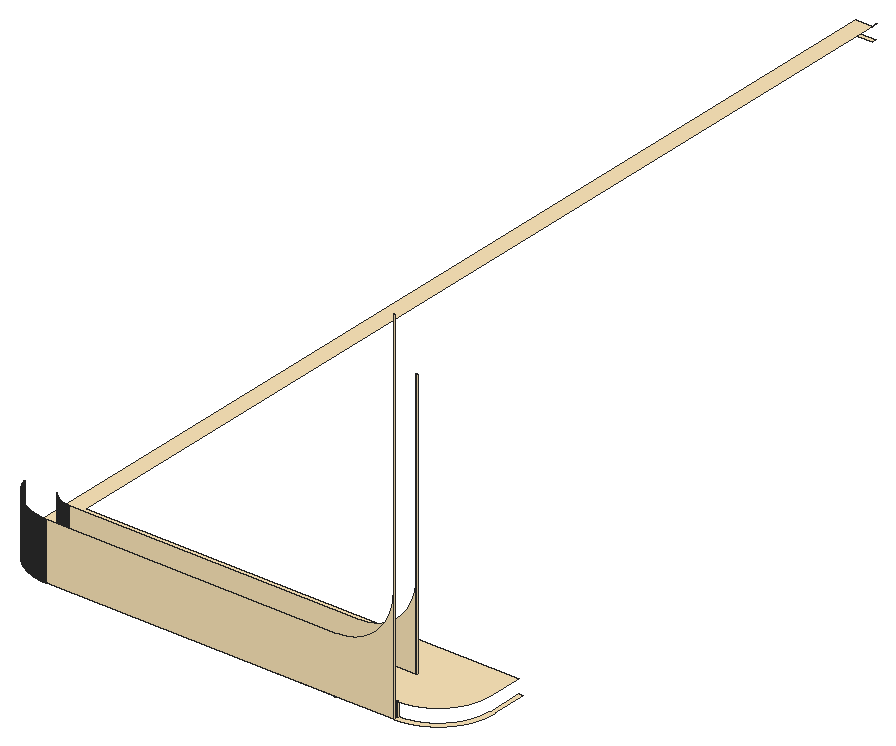
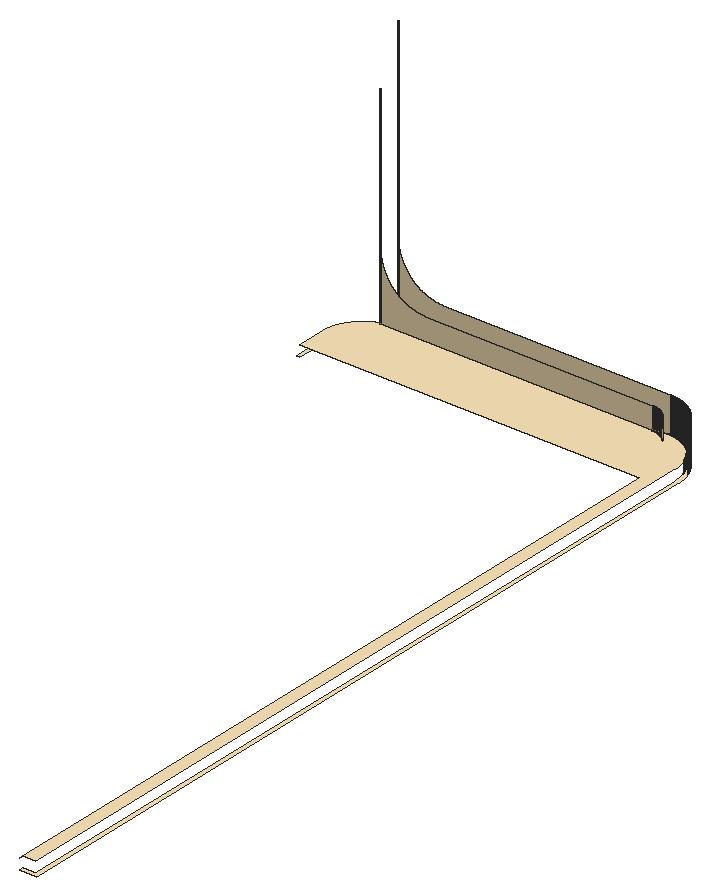
# SketchUp Ruby script. Lengths in inches.
U = 1.inch
M = Sketchup.active_model
def pt(a) = Geom::Point3d.new(a.map { |v| v * U })
def face(e, loops, mat)
  f = e.add_face(loops[0].map { |a| pt(a) })
  loops[1..].each { |l| e.add_face(l.map { |a| pt(a) }).erase! }
  f.material = f.back_material = mat if mat
  f
end
# faces: each face lists its corners as indices into pts; further lists are holes
def faces(e, pts, list, mat = nil) = list.each { |f| face(e, (f[0].is_a?(Array) ? f : [f]).map { |l| l.map { |i| pts[i] } }, mat) }
# xy, xz, yz: faces in a plane at the given z, y or x. An outline is a flat list of corners, or four numbers for a rectangle; further outlines are holes
def ring(l) = l.size == 4 ? [[l[0], l[1]], [l[2], l[1]], [l[2], l[3]], [l[0], l[3]]] : l.each_slice(2).to_a
def flat(e, list, mat, &to3) = list.each { |f| face(e, (f[0].is_a?(Array) ? f : [f]).map { |l| ring(l).map { |u, v| to3.(u, v) } }, mat) }
def xy(e, z, list, mat = nil) = flat(e, list, mat) { |x, y| [x, y, z] }
def xz(e, y, list, mat = nil) = flat(e, list, mat) { |x, z| [x, y, z] }
def yz(e, x, list, mat = nil) = flat(e, list, mat) { |y, z| [x, y, z] }
def lines(e, pts, list) = list.each { |a, b| e.add_line(pt(pts[a]), pt(pts[b])) }
# prism: a flat outline (further loops are holes) pulled along v
def prism(e, loops, v, mat = nil)
  f = face(e, loops, mat); d = Geom::Vector3d.new(v.map { |x| x * U })
  f.pushpull(f.normal.samedirection?(d) ? d.length : -d.length)
end
def box(e, o, s, mat = nil) = prism(e, [[o, [o[0] + s[0], o[1], o[2]], [o[0] + s[0], o[1] + s[1], o[2]], [o[0], o[1] + s[1], o[2]]]], [0, 0, s[2]], mat)
def at(x, y, z, deg = 0) = Geom::Transformation.translation(pt([x, y, z])) * Geom::Transformation.rotation(ORIGIN, Z_AXIS, deg.degrees)
def axes(o, x, y, z) = Geom::Transformation.new([*x, 0, *y, 0, *z, 0, *pt(o).to_a, 1])
def part(name) = M.definitions.add(name)
# library, detail: a bought-in or finely detailed component or shape, given as its bounding box
def library(name, o, s) = part(name).tap { |d| box(d.entities, o, s) }
def detail(e, o, s) = box(e.add_group.entities, o, s)
def put(e, d, t, mat = nil) = e.add_instance(d, t).tap { |i| i.material = mat if mat }
def group(e, t, mat = nil) = e.add_group.tap { |g| g.transformation = t; g.material = mat if mat }.entities
root = M.entities
M.materials.add("1026 AP 7946 SUNNY SIDE UP").color = [254, 231, 186]
xy(root,120,[[153,215,29.765,215.001,29.529,215.005,29.294,215.01,29.059,215.018,28.824,215.029,28.589,215.041,28.354,215.056,28.119,215.074,27.885,215.093,27.65,215.115,27.416,215.139,27.182,215.166,26.949,215.195,26.715,215.226,26.483,215.259,26.25,215.295,26.018,215.333,25.786,215.373,25.554,215.415,25.323,215.46,25.093,215.507,24.862,215.556,24.633,215.608,24.404,215.661,24.175,215.717,23.947,215.776,23.72,215.836,23.493,215.899,23.267,215.964,23.041,216.031,22.816,216.1,22.592,216.172,22.368,216.246,22.146,216.321,21.924,216.4,21.702,216.48,21.482,216.562,21.262,216.647,21.044,216.734,20.826,216.823,20.609,216.914,20.392,217.007,20.177,217.102,19.963,217.199,19.75,217.299,19.537,217.4,19.326,217.504,19.116,217.61,18.907,217.717,18.698,217.827,18.491,217.939,18.285,218.053,18.081,218.169,17.877,218.287,17.674,218.407,17.473,218.528,17.273,218.652,17.074,218.778,16.876,218.906,16.68,219.035,16.485,219.167,16.291,219.3,16.098,219.436,15.907,219.573,15.717,219.712,15.529,219.853,15.342,219.996,15.156,220.141,14.972,220.287,14.789,220.435,14.608,220.585,14.428,220.737,14.25,220.891,14.073,221.046,13.898,221.203,13.724,221.362,13.552,221.522,13.381,221.684,13.212,221.848,13.045,222.014,12.879,222.181,12.715,222.349,12.552,222.52,12.392,222.692,12.233,222.865,12.075,223.04,11.92,223.217,11.766,223.395,11.614,223.574,11.463,223.755,11.315,223.9375,11.168,224.122,11.023,224.307,10.88,224.494,10.738,224.682,10.599,224.872,10.461,225.0625,10.325,225.255,10.192,225.448,10.06,225.643,9.93,225.839,9.802,226.037,9.675,226.235,9.551,226.435,9.429,226.637,9.309,226.839,9.19,227.042,9.074,227.247,8.96,227.453,8.848,227.66,8.738,227.868,8.629,228.077,8.523,228.287,8.419,228.498,8.317,228.71,8.218,228.923,8.12,229.137,8.024,229.352,7.931,229.568,7.839,229.785,7.75,230.003,7.663,230.221,7.578,230.441,7.495,230.661,7.414,230.882,7.336,231.104,7.259,231.327,7.185,231.55,7.113,231.774,7.043,231.999,6.976,232.224,6.91,232.45,6.847,232.677,6.786,232.904,6.728,233.132,6.671,233.361,6.617,233.59,6.565,233.819,6.516,234.049,6.468,234.28,6.423,234.511,6.38,234.742,6.34,234.974,6.301,235.206,6.265,235.439,6.231,235.672,6.2,235.905,6.171,236.138,6.144,236.372,6.119,236.606,6.097,236.841,6.077,237.075,6.059,237.31,6.044,237.545,6.031,237.78,6.02,238.015,6.011,238.25,6.005,238.485,6.001,238.72,5.999,238.956,6,239,6,674,15,674,15,672,8,672,8,238.989,7.999,238.96,8.001,238.744,8.005,238.528,8.01,238.3125,8.018,238.097,8.028,237.881,8.04,237.666,8.054,237.451,8.07,237.236,8.089,237.021,8.109,236.806,8.132,236.591,8.156,236.377,8.183,236.163,8.212,235.949,8.243,235.736,8.276,235.522,8.311,235.31,8.348,235.097,8.388,234.885,8.429,234.673,8.473,234.462,8.518,234.251,8.566,234.041,8.615,233.831,8.667,233.621,8.721,233.412,8.777,233.204,8.835,232.996,8.894,232.789,8.956,232.582,9.02,232.376,9.086,232.171,9.154,231.966,9.224,231.762,9.296,231.559,9.37,231.356,9.446,231.154,9.524,230.953,9.604,230.752,9.686,230.553,9.77,230.354,9.855,230.156,9.943,229.959,10.033,229.763,10.124,229.567,10.218,229.373,10.313,229.179,10.41,228.987,10.509,228.795,10.61,228.605,10.713,228.415,10.818,228.226,10.925,228.039,11.033,227.852,11.143,227.667,11.255,227.482,11.369,227.299,11.485,227.117,11.602,226.936,11.721,226.756,11.842,226.578,11.965,226.4,12.089,226.224,12.215,226.049,12.343,225.875,12.473,225.703,12.604,225.531,12.737,225.361,12.872,225.193,13.008,225.026,13.146,224.86,13.285,224.695,13.426,224.532,13.569,224.37,13.713,224.21,13.859,224.051,14.006,223.893,14.155,223.737,14.306,223.582,14.458,223.429,14.611,223.278,14.766,223.127,14.922,222.979,15.08,222.832,15.239,222.686,15.4,222.542,15.562,222.4,15.726,222.259,15.891,222.12,16.057,221.982,16.224,221.846,16.393,221.712,16.563,221.58,16.735,221.449,16.908,221.319,17.082,221.192,17.257,221.066,17.433,220.942,17.611,220.82,17.79,220.699,17.97,220.58,18.151,220.463,18.333,220.348,18.517,220.234,18.701,220.123,18.887,220.013,19.074,219.905,19.262,219.798,19.45,219.694,19.64,219.592,19.831,219.491,20.023,219.392,20.216,219.295,20.409,219.2,20.604,219.107,20.799,219.016,20.996,218.927,21.193,218.839,21.391,218.754,21.59,218.671,21.79,218.589,21.99,218.51,22.192,218.432,22.394,218.357,22.597,218.283,22.8,218.211,23.004,218.142,23.209,218.074,23.415,218.009,23.621,217.945,23.828,217.883,24.035,217.824,24.243,217.766,24.451,217.711,24.66,217.658,24.87,217.606,25.08,217.557,25.291,217.51,25.501,217.465,25.713,217.422,25.925,217.381,26.137,217.342,26.349,217.305,26.5625,217.27,26.776,217.237,26.989,217.207,27.203,217.178,27.417,217.152,27.631,217.128,27.846,217.106,28.061,217.086,28.276,217.068,28.491,217.052,28.706,217.038,28.922,217.026,29.137,217.017,29.353,217.01,29.569,217.004,29.784,217.001,153,217,177,217,177.23,217.001,177.461,217.005,177.691,217.011,177.921,217.019,178.151,217.03,178.381,217.043,178.611,217.059,178.841,217.077,179.07,217.098,179.3,217.121,179.529,217.146,179.757,217.173,179.986,217.204,180.214,217.236,180.442,217.271,180.669,217.308,180.896,217.348,181.122,217.39,181.348,217.434,181.574,217.481,181.799,217.53,182.024,217.581,182.248,217.635,182.471,217.691,182.694,217.75,182.916,217.81,183.138,217.874,183.359,217.939,183.579,218.007,183.798,218.077,184.017,218.149,184.235,218.224,184.452,218.301,184.669,218.38,184.884,218.461,185.099,218.545,185.3125,218.631,185.525,218.719,185.737,218.809,185.948,218.902,186.158,218.997,186.367,219.094,186.575,219.193,186.782,219.294,186.988,219.398,187.193,219.504,187.396,219.611,187.599,219.721,187.8,219.833,188,219.947,188.199,220.064,188.397,220.182,188.593,220.302,188.788,220.425,188.982,220.549,189.175,220.676,189.366,220.804,189.556,220.935,189.744,221.067,189.931,221.202,190.117,221.338,190.301,221.476,190.484,221.617,190.665,221.759,190.845,221.903,191.023,222.049,191.2,222.196,191.375,222.346,191.549,222.498,191.721,222.651,191.891,222.806,192.06,222.963,192.227,223.121,192.393,223.282,192.556,223.444,192.718,223.607,192.879,223.773,193.037,223.94,193.194,224.109,193.349,224.279,193.502,224.451,193.654,224.625,193.804,224.8,193.951,224.977,194.097,225.155,194.241,225.335,194.383,225.516,194.524,225.699,194.662,225.883,194.798,226.069,194.933,226.256,195.065,226.444,195.196,226.634,195.324,226.825,195.451,227.018,195.575,227.212,195.698,227.407,195.818,227.603,195.936,227.801,196.053,228,196.167,228.2,196.279,228.401,196.389,228.604,196.496,228.807,196.602,229.012,196.706,229.218,196.807,229.425,196.906,229.633,197.003,229.842,197.098,230.052,197.191,230.263,197.281,230.475,197.369,230.6875,197.455,230.901,197.539,231.116,197.62,231.331,197.699,231.548,197.776,231.765,197.851,231.983,197.923,232.202,197.993,232.421,198.061,232.641,198.126,232.862,198.19,233.084,198.25,233.306,198.309,233.529,198.365,233.752,198.419,233.976,198.47,234.201,198.519,234.426,198.566,234.652,198.61,234.878,198.652,235.104,198.692,235.331,198.729,235.558,198.764,235.786,198.796,236.014,198.827,236.243,198.854,236.471,198.879,236.7,198.902,236.93,198.923,237.159,198.941,237.389,198.957,237.619,198.97,237.849,198.981,238.079,198.989,238.309,198.995,238.539,198.999,238.77,199,239,199,254,201,254,201,239,200.999,238.749,200.995,238.497,200.988,238.246,200.979,237.995,200.967,237.744,200.953,237.493,200.936,237.242,200.916,236.992,200.893,236.741,200.869,236.491,200.841,236.242,200.811,235.992,200.778,235.743,200.743,235.494,200.705,235.246,200.664,234.998,200.621,234.75,200.575,234.503,200.527,234.256,200.476,234.01,200.422,233.765,200.366,233.52,200.307,233.275,200.246,233.031,200.182,232.788,200.116,232.546,200.047,232.304,199.976,232.063,199.902,231.823,199.825,231.584,199.746,231.345,199.665,231.107,199.581,230.87,199.495,230.634,199.406,230.399,199.315,230.165,199.221,229.932,199.125,229.7,199.026,229.468,198.925,229.238,198.822,229.009,198.716,228.781,198.608,228.554,198.497,228.329,198.384,228.104,198.269,227.881,198.151,227.659,198.031,227.438,197.909,227.218,197.785,227,197.658,226.783,197.529,226.567,197.397,226.353,197.264,226.14,197.128,225.929,196.99,225.719,196.85,225.51,196.708,225.303,196.563,225.097,196.416,224.893,196.268,224.691,196.117,224.49,195.964,224.29,195.809,224.092,195.652,223.896,195.492,223.702,195.331,223.509,195.168,223.318,195.003,223.129,194.835,222.941,194.666,222.755,194.495,222.571,194.322,222.389,194.147,222.208,193.971,222.029,193.792,221.853,193.611,221.678,193.429,221.505,193.245,221.334,193.059,221.165,192.871,220.997,192.682,220.832,192.491,220.669,192.298,220.508,192.104,220.348,191.908,220.191,191.71,220.036,191.51,219.883,191.309,219.732,191.107,219.584,190.903,219.437,190.697,219.292,190.49,219.15,190.281,219.01,190.071,218.872,189.86,218.736,189.647,218.603,189.433,218.471,189.217,218.342,189,218.215,188.782,218.091,188.562,217.969,188.341,217.849,188.119,217.731,187.896,217.616,187.671,217.503,187.446,217.392,187.219,217.284,186.991,217.178,186.762,217.075,186.532,216.974,186.3,216.875,186.068,216.779,185.835,216.685,185.601,216.594,185.366,216.505,185.13,216.419,184.893,216.335,184.655,216.254,184.416,216.175,184.177,216.098,183.937,216.024,183.696,215.953,183.454,215.884,183.212,215.818,182.969,215.754,182.725,215.693,182.48,215.634,182.235,215.578,181.99,215.524,181.744,215.473,181.497,215.425,181.25,215.379,181.002,215.336,180.754,215.295,180.506,215.257,180.257,215.222,180.008,215.189,179.758,215.159,179.509,215.131,179.259,215.107,179.008,215.084,178.758,215.064,178.507,215.047,178.256,215.033,178.005,215.021,177.754,215.012,177.503,215.005,177.251,215.001,177,215],[30,215,29.765,215.001,153,215]],"1026 AP 7946 SUNNY SIDE UP")
xy(root,126,[[153,217,29.784,217.001,29.569,217.004,29.353,217.01,29.137,217.017,28.922,217.026,28.706,217.038,28.491,217.052,28.276,217.068,28.061,217.086,27.846,217.106,27.631,217.128,27.417,217.152,27.203,217.178,26.989,217.207,26.776,217.237,26.5625,217.27,26.349,217.305,26.137,217.342,25.925,217.381,25.713,217.422,25.501,217.465,25.291,217.51,25.08,217.557,24.87,217.606,24.66,217.658,24.451,217.711,24.243,217.766,24.035,217.824,23.828,217.883,23.621,217.945,23.415,218.009,23.209,218.074,23.004,218.142,22.8,218.211,22.597,218.283,22.394,218.357,22.192,218.432,21.99,218.51,21.79,218.589,21.59,218.671,21.391,218.754,21.193,218.839,20.996,218.927,20.799,219.016,20.604,219.107,20.409,219.2,20.216,219.295,20.023,219.392,19.831,219.491,19.64,219.592,19.45,219.694,19.262,219.798,19.074,219.905,18.887,220.013,18.701,220.123,18.517,220.234,18.333,220.348,18.151,220.463,17.97,220.58,17.79,220.699,17.611,220.82,17.433,220.942,17.257,221.066,17.082,221.192,16.908,221.319,16.735,221.449,16.563,221.58,16.393,221.712,16.224,221.846,16.057,221.982,15.891,222.12,15.726,222.259,15.562,222.4,15.4,222.542,15.239,222.686,15.08,222.832,14.922,222.979,14.766,223.127,14.611,223.278,14.458,223.429,14.306,223.582,14.155,223.737,14.006,223.893,13.859,224.051,13.713,224.21,13.569,224.37,13.426,224.532,13.285,224.695,13.146,224.86,13.008,225.026,12.872,225.193,12.737,225.361,12.604,225.531,12.473,225.703,12.343,225.875,12.215,226.049,12.089,226.224,11.965,226.4,11.842,226.578,11.721,226.756,11.602,226.936,11.485,227.117,11.369,227.299,11.255,227.482,11.143,227.667,11.033,227.852,10.925,228.039,10.818,228.226,10.713,228.415,10.61,228.605,10.509,228.795,10.41,228.987,10.313,229.179,10.218,229.373,10.124,229.567,10.033,229.763,9.943,229.959,9.855,230.156,9.77,230.354,9.686,230.553,9.604,230.752,9.524,230.953,9.446,231.154,9.37,231.356,9.296,231.559,9.224,231.762,9.154,231.966,9.086,232.171,9.02,232.376,8.956,232.582,8.894,232.789,8.835,232.996,8.777,233.204,8.721,233.412,8.667,233.621,8.615,233.831,8.566,234.041,8.518,234.251,8.473,234.462,8.429,234.673,8.388,234.885,8.348,235.097,8.311,235.31,8.276,235.522,8.243,235.736,8.212,235.949,8.183,236.163,8.156,236.377,8.132,236.591,8.109,236.806,8.089,237.021,8.07,237.236,8.054,237.451,8.04,237.666,8.028,237.881,8.018,238.097,8.01,238.3125,8.005,238.528,8.001,238.744,7.999,238.96,8,238.989,8,672,15,672,15,674,15.035,674,15.035,254,199,254,199,239,198.999,238.77,198.995,238.539,198.989,238.309,198.981,238.079,198.97,237.849,198.957,237.619,198.941,237.389,198.923,237.159,198.902,236.93,198.879,236.7,198.854,236.471,198.827,236.243,198.796,236.014,198.764,235.786,198.729,235.558,198.692,235.331,198.652,235.104,198.61,234.878,198.566,234.652,198.519,234.426,198.47,234.201,198.419,233.976,198.365,233.752,198.309,233.529,198.25,233.306,198.19,233.084,198.126,232.862,198.061,232.641,197.993,232.421,197.923,232.202,197.851,231.983,197.776,231.765,197.699,231.548,197.62,231.331,197.539,231.116,197.455,230.901,197.369,230.6875,197.281,230.475,197.191,230.263,197.098,230.052,197.003,229.842,196.906,229.633,196.807,229.425,196.706,229.218,196.602,229.012,196.496,228.807,196.389,228.604,196.279,228.401,196.167,228.2,196.053,228,195.936,227.801,195.818,227.603,195.698,227.407,195.575,227.212,195.451,227.018,195.324,226.825,195.196,226.634,195.065,226.444,194.933,226.256,194.798,226.069,194.662,225.883,194.524,225.699,194.383,225.516,194.241,225.335,194.097,225.155,193.951,224.977,193.804,224.8,193.654,224.625,193.502,224.451,193.349,224.279,193.194,224.109,193.037,223.94,192.879,223.773,192.718,223.607,192.556,223.444,192.393,223.282,192.227,223.121,192.06,222.963,191.891,222.806,191.721,222.651,191.549,222.498,191.375,222.346,191.2,222.196,191.023,222.049,190.845,221.903,190.665,221.759,190.484,221.617,190.301,221.476,190.117,221.338,189.931,221.202,189.744,221.067,189.556,220.935,189.366,220.804,189.175,220.676,188.982,220.549,188.788,220.425,188.593,220.302,188.397,220.182,188.199,220.064,188,219.947,187.8,219.833,187.599,219.721,187.396,219.611,187.193,219.504,186.988,219.398,186.782,219.294,186.575,219.193,186.367,219.094,186.158,218.997,185.948,218.902,185.737,218.809,185.525,218.719,185.3125,218.631,185.099,218.545,184.884,218.461,184.669,218.38,184.452,218.301,184.235,218.224,184.017,218.149,183.798,218.077,183.579,218.007,183.359,217.939,183.138,217.874,182.916,217.81,182.694,217.75,182.471,217.691,182.248,217.635,182.024,217.581,181.799,217.53,181.574,217.481,181.348,217.434,181.122,217.39,180.896,217.348,180.669,217.308,180.442,217.271,180.214,217.236,179.986,217.204,179.757,217.173,179.529,217.146,179.3,217.121,179.07,217.098,178.841,217.077,178.611,217.059,178.381,217.043,178.151,217.03,177.921,217.019,177.691,217.011,177.461,217.005,177.23,217.001,177,217]],"1026 AP 7946 SUNNY SIDE UP")
xz(root,217,[[153,120,177,126]],"1026 AP 7946 SUNNY SIDE UP")
xz(root,227,[[30,132,30,144,153,144,153.236,144.001,153.471,144.005,153.707,144.01,153.942,144.019,154.178,144.029,154.413,144.042,154.648,144.057,154.883,144.074,155.118,144.094,155.352,144.116,155.587,144.14,155.821,144.166,156.055,144.195,156.288,144.226,156.522,144.26,156.754,144.295,156.987,144.333,157.219,144.374,157.451,144.416,157.682,144.461,157.913,144.508,158.143,144.558,158.373,144.609,158.603,144.663,158.832,144.719,159.06,144.778,159.287,144.838,159.515,144.901,159.741,144.966,159.967,145.033,160.192,145.103,160.416,145.175,160.64,145.249,160.863,145.325,161.085,145.403,161.307,145.483,161.527,145.566,161.747,145.651,161.966,145.738,162.184,145.827,162.402,145.918,162.618,146.011,162.833,146.107,163.048,146.205,163.261,146.304,163.474,146.406,163.685,146.51,163.896,146.616,164.105,146.724,164.314,146.834,164.521,146.946,164.727,147.06,164.932,147.176,165.136,147.294,165.338,147.415,165.54,147.537,165.74,147.661,165.939,147.787,166.137,147.915,166.334,148.045,166.529,148.177,166.723,148.31,166.916,148.446,167.107,148.584,167.297,148.723,167.485,148.864,167.673,149.007,167.858,149.152,168.043,149.299,168.225,149.448,168.407,149.598,168.587,149.75,168.765,149.904,168.942,150.06,169.117,150.217,169.291,150.376,169.463,150.537,169.634,150.7,169.803,150.864,169.971,151.029,170.136,151.197,170.3,151.366,170.463,151.537,170.624,151.709,170.783,151.883,170.94,152.058,171.096,152.235,171.25,152.413,171.402,152.593,171.552,152.775,171.701,152.957,171.848,153.142,171.993,153.327,172.136,153.515,172.277,153.703,172.416,153.893,172.554,154.084,172.69,154.277,172.823,154.471,172.955,154.666,173.085,154.863,173.213,155.061,173.339,155.26,173.463,155.46,173.585,155.662,173.706,155.864,173.824,156.068,173.94,156.273,174.054,156.479,174.166,156.686,174.276,156.895,174.384,157.104,174.49,157.315,174.594,157.526,174.696,157.739,174.795,157.952,174.893,158.167,174.989,158.382,175.082,158.598,175.173,158.816,175.262,159.034,175.349,159.253,175.434,159.473,175.517,159.693,175.597,159.915,175.675,160.137,175.751,160.36,175.825,160.584,175.897,160.808,175.967,161.033,176.034,161.259,176.099,161.485,176.162,161.713,176.222,161.94,176.281,162.168,176.337,162.397,176.391,162.627,176.442,162.857,176.492,163.087,176.539,163.318,176.584,163.549,176.626,163.781,176.667,164.013,176.705,164.246,176.74,164.478,176.774,164.712,176.805,164.945,176.834,165.179,176.86,165.413,176.884,165.648,176.906,165.882,176.926,166.117,176.943,166.352,176.958,166.587,176.971,166.822,176.981,167.058,176.99,167.293,176.995,167.529,176.999,167.764,177,168,177,132]],"1026 AP 7946 SUNNY SIDE UP")
p = [[28.354,215.056,120],[28.589,215.041,120],[28.589,215.041,144],[28.354,215.056,144],[28.824,215.029,120],[28.824,215.029,144],
  [29.059,215.018,120],[29.059,215.018,144],[29.294,215.01,120],[29.294,215.01,144],[29.529,215.005,120],[29.529,215.005,144],
  [29.765,215.001,120],[29.765,215.001,142],[29.765,215.001,144],[153,215,120],[177,215,120],[177,215,168],
  [176.999,215,167.764],[176.995,215,167.529],[176.99,215,167.293],[176.981,215,167.058],[176.971,215,166.822],[176.958,215,166.587],
  [176.943,215,166.352],[176.926,215,166.117],[176.906,215,165.882],[176.884,215,165.648],[176.86,215,165.413],[176.834,215,165.179],
  [176.805,215,164.945],[176.774,215,164.712],[176.74,215,164.478],[176.705,215,164.246],[176.667,215,164.013],[176.626,215,163.781],
  [176.584,215,163.549],[176.539,215,163.318],[176.492,215,163.087],[176.442,215,162.857],[176.391,215,162.627],[176.337,215,162.397],
  [176.281,215,162.168],[176.222,215,161.94],[176.162,215,161.713],[176.099,215,161.485],[176.034,215,161.259],[175.967,215,161.033],
  [175.897,215,160.808],[175.825,215,160.584],[175.751,215,160.36],[175.675,215,160.137],[175.597,215,159.915],[175.517,215,159.693],
  [175.434,215,159.473],[175.349,215,159.253],[175.262,215,159.034],[175.173,215,158.816],[175.082,215,158.598],[174.989,215,158.382],
  [174.893,215,158.167],[174.795,215,157.952],[174.696,215,157.739],[174.594,215,157.526],[174.49,215,157.315],[174.384,215,157.104],
  [174.276,215,156.895],[174.166,215,156.686],[174.054,215,156.479],[173.94,215,156.273],[173.824,215,156.068],[173.706,215,155.864],
  [173.585,215,155.662],[173.463,215,155.46],[173.339,215,155.26],[173.213,215,155.061],[173.085,215,154.863],[172.955,215,154.666],
  [172.823,215,154.471],[172.69,215,154.277],[172.554,215,154.084],[172.416,215,153.893],[172.277,215,153.703],[172.136,215,153.515],
  [171.993,215,153.327],[171.848,215,153.142],[171.701,215,152.957],[171.552,215,152.775],[171.402,215,152.593],[171.25,215,152.413],
  [171.096,215,152.235],[170.94,215,152.058],[170.783,215,151.883],[170.624,215,151.709],[170.463,215,151.537],[170.3,215,151.366],
  [170.136,215,151.197],[169.971,215,151.029],[169.803,215,150.864],[169.634,215,150.7],[169.463,215,150.537],[169.291,215,150.376],
  [169.117,215,150.217],[168.942,215,150.06],[168.765,215,149.904],[168.587,215,149.75],[168.407,215,149.598],[168.225,215,149.448],
  [168.043,215,149.299],[167.858,215,149.152],[167.673,215,149.007],[167.485,215,148.864],[167.297,215,148.723],[167.107,215,148.584],
  [166.916,215,148.446],[166.723,215,148.31],[166.529,215,148.177],[166.334,215,148.045],[166.137,215,147.915],[165.939,215,147.787],
  [165.74,215,147.661],[165.54,215,147.537],[165.338,215,147.415],[165.136,215,147.294],[164.932,215,147.176],[164.727,215,147.06],
  [164.521,215,146.946],[164.314,215,146.834],[164.105,215,146.724],[163.896,215,146.616],[163.685,215,146.51],[163.474,215,146.406],
  [163.261,215,146.304],[163.048,215,146.205],[162.833,215,146.107],[162.618,215,146.011],[162.402,215,145.918],[162.184,215,145.827],
  [161.966,215,145.738],[161.747,215,145.651],[161.527,215,145.566],[161.307,215,145.483],[161.085,215,145.403],[160.863,215,145.325],
  [160.64,215,145.249],[160.416,215,145.175],[160.192,215,145.103],[159.967,215,145.033],[159.741,215,144.966],[159.515,215,144.901],
  [159.287,215,144.838],[159.06,215,144.778],[158.832,215,144.719],[158.603,215,144.663],[158.373,215,144.609],[158.143,215,144.558],
  [157.913,215,144.508],[157.682,215,144.461],[157.451,215,144.416],[157.219,215,144.374],[156.987,215,144.333],[156.754,215,144.295],
  [156.522,215,144.26],[156.288,215,144.226],[156.055,215,144.195],[155.821,215,144.166],[155.587,215,144.14],[155.352,215,144.116],
  [155.118,215,144.094],[154.883,215,144.074],[154.648,215,144.057],[154.413,215,144.042],[154.178,215,144.029],[153.942,215,144.019],
  [153.707,215,144.01],[153.471,215,144.005],[153.236,215,144.001],[153.231,215,144.001],[153,215,144],[30,215.001,144],
  [177.251,215.001,120],[177.251,215.001,274],[177,215,274],[177,215,222],[177.503,215.005,120],[177.503,215.005,274],
  [27.182,215.166,120],[27.416,215.139,120],[27.416,215.139,144],[27.182,215.166,144],[27.65,215.115,120],[27.65,215.115,144],
  [27.885,215.093,120],[27.885,215.093,144],[28.119,215.074,120],[28.119,215.074,144],[26.483,215.259,120],[26.715,215.226,120],
  [26.715,215.226,144],[26.483,215.259,144],[26.949,215.195,120],[26.949,215.195,144],[25.786,215.373,120],[26.018,215.333,120],
  [26.018,215.333,144],[25.786,215.373,144],[26.25,215.295,120],[26.25,215.295,144],[25.323,215.46,120],[25.554,215.415,120],
  [25.554,215.415,144],[25.323,215.46,144],[24.862,215.556,120],[25.093,215.507,120],[25.093,215.507,144],[24.862,215.556,144],
  [24.404,215.661,120],[24.633,215.608,120],[24.633,215.608,144],[24.404,215.661,144],[23.947,215.776,120],[24.175,215.717,120],
  [24.175,215.717,144],[23.947,215.776,144],[23.493,215.899,120],[23.72,215.836,120],[23.72,215.836,144],[23.493,215.899,144],
  [23.267,215.964,120],[23.267,215.964,144],[22.816,216.1,120],[23.041,216.031,120],[23.041,216.031,144],[22.816,216.1,144],
  [22.592,216.172,120],[22.592,216.172,144],[22.146,216.321,120],[22.368,216.246,120],[22.368,216.246,144],[22.146,216.321,144],
  [21.924,216.4,120],[21.924,216.4,144],[21.702,216.48,120],[21.702,216.48,144],[21.482,216.562,120],[21.482,216.562,144],
  [21.044,216.734,120],[21.262,216.647,120],[21.262,216.647,144],[21.044,216.734,144],[20.826,216.823,120],[20.826,216.823,144],
  [20.609,216.914,120],[20.609,216.914,144],[20.392,217.007,120],[20.392,217.007,144],[20.177,217.102,120],[20.177,217.102,144],
  [28.706,217.038,120],[28.491,217.052,120],[28.491,217.052,126],[28.706,217.038,126],[28.922,217.026,120],[28.922,217.026,126],
  [29.137,217.017,120],[29.137,217.017,126],[29.353,217.01,120],[29.353,217.01,126],[29.569,217.004,120],[29.569,217.004,126],
  [29.784,217.001,120],[29.784,217.001,126],[153,217,120],[153,217,126],[177.23,217.001,120],[177,217,120],
  [177,217,126],[177.23,217.001,126],[177.461,217.005,120],[177.461,217.005,126],[177.691,217.011,120],[177.691,217.011,126],
  [19.963,217.199,120],[19.963,217.199,144],[27.631,217.128,120],[27.417,217.152,120],[27.417,217.152,126],[27.631,217.128,126],
  [27.846,217.106,120],[27.846,217.106,126],[28.061,217.086,120],[28.061,217.086,126],[28.276,217.068,120],[28.276,217.068,126],
  [19.75,217.299,120],[19.75,217.299,144],[26.776,217.237,120],[26.5625,217.27,120],[26.5625,217.27,126],[26.776,217.237,126],
  [26.989,217.207,120],[26.989,217.207,126],[27.203,217.178,120],[27.203,217.178,126],[19.537,217.4,120],[19.537,217.4,144],
  [26.137,217.342,120],[25.925,217.381,120],[25.925,217.381,126],[26.137,217.342,126],[26.349,217.305,120],[26.349,217.305,126],
  [19.326,217.504,120],[19.326,217.504,144],[25.713,217.422,120],[25.501,217.465,120],[25.501,217.465,126],[25.713,217.422,126],
  [19.116,217.61,120],[19.116,217.61,144],[25.291,217.51,120],[25.08,217.557,120],[25.08,217.557,126],[25.291,217.51,126],
  [18.907,217.717,120],[18.907,217.717,144],[24.87,217.606,120],[24.66,217.658,120],[24.66,217.658,126],[24.87,217.606,126],
  [18.698,217.827,120],[18.698,217.827,144],[24.451,217.711,120],[24.243,217.766,120],[24.243,217.766,126],[24.451,217.711,126],
  [18.491,217.939,120],[18.491,217.939,144],[24.035,217.824,120],[23.828,217.883,120],[23.828,217.883,126],[24.035,217.824,126],
  [18.285,218.053,120],[18.285,218.053,144],[23.621,217.945,120],[23.415,218.009,120],[23.415,218.009,126],[23.621,217.945,126],
  [23.209,218.074,120],[23.209,218.074,126],[18.081,218.169,120],[18.081,218.169,144],[23.004,218.142,120],[22.8,218.211,120],
  [22.8,218.211,126],[23.004,218.142,126],[17.877,218.287,120],[17.877,218.287,144],[22.597,218.283,120],[22.597,218.283,126],
  [17.674,218.407,120],[17.674,218.407,144],[22.394,218.357,120],[22.394,218.357,126],[17.473,218.528,120],[17.473,218.528,144],
  [22.192,218.432,120],[21.99,218.51,120],[21.99,218.51,126],[22.192,218.432,126],[17.273,218.652,120],[17.273,218.652,144],
  [21.79,218.589,120],[21.79,218.589,126],[21.59,218.671,120],[21.59,218.671,126],[17.074,218.778,120],[17.074,218.778,144],
  [21.391,218.754,120],[21.391,218.754,126],[16.876,218.906,120],[16.876,218.906,144],[21.193,218.839,120],[20.996,218.927,120],
  [20.996,218.927,126],[21.193,218.839,126],[16.68,219.035,120],[16.68,219.035,144],[20.799,219.016,120],[20.799,219.016,126],
  [16.485,219.167,120],[16.485,219.167,144],[20.604,219.107,120],[20.604,219.107,126],[20.409,219.2,120],[20.409,219.2,126],
  [16.291,219.3,120],[16.291,219.3,144],[20.216,219.295,120],[20.216,219.295,126],[16.098,219.436,120],[16.098,219.436,144],
  [20.023,219.392,120],[20.023,219.392,126],[15.907,219.573,120],[15.907,219.573,144],[19.831,219.491,120],[19.831,219.491,126],
  [19.64,219.592,120],[19.64,219.592,126],[15.717,219.712,120],[15.717,219.712,144],[19.45,219.694,120],[19.45,219.694,126],
  [15.529,219.853,120],[15.529,219.853,144],[19.262,219.798,120],[19.262,219.798,126],[19.074,219.905,120],[19.074,219.905,126],
  [15.342,219.996,120],[15.342,219.996,144],[18.887,220.013,120],[18.887,220.013,126],[15.156,220.141,120],[15.156,220.141,144],
  [18.701,220.123,120],[18.701,220.123,126],[14.972,220.287,120],[14.972,220.287,144],[18.517,220.234,120],[18.517,220.234,126],
  [18.333,220.348,120],[18.333,220.348,126],[14.789,220.435,120],[14.789,220.435,144],[18.151,220.463,120],[18.151,220.463,126],
  [14.608,220.585,120],[14.608,220.585,144],[17.97,220.58,120],[17.97,220.58,126],[14.428,220.737,120],[14.428,220.737,144],
  [17.79,220.699,120],[17.79,220.699,126],[14.25,220.891,120],[14.25,220.891,144],[17.611,220.82,120],[17.611,220.82,126],
  [17.433,220.942,120],[17.433,220.942,126],[14.073,221.046,120],[14.073,221.046,144],[17.257,221.066,120],[17.257,221.066,126],
  [13.898,221.203,120],[13.898,221.203,144],[17.082,221.192,120],[17.082,221.192,126],[13.724,221.362,120],[13.724,221.362,144],
  [16.908,221.319,120],[16.908,221.319,126],[16.735,221.449,120],[16.735,221.449,126],[13.552,221.522,120],[13.552,221.522,144],
  [16.563,221.58,120],[16.563,221.58,126],[13.381,221.684,120],[13.381,221.684,144],[16.393,221.712,120],[16.393,221.712,126],
  [13.212,221.848,120],[13.212,221.848,144],[16.224,221.846,120],[16.224,221.846,126],[13.045,222.014,120],[13.045,222.014,144],
  [16.057,221.982,120],[16.057,221.982,126],[12.879,222.181,120],[12.879,222.181,144],[15.891,222.12,120],[15.891,222.12,126],
  [15.726,222.259,120],[15.726,222.259,126],[12.715,222.349,120],[12.715,222.349,144],[12.552,222.52,120],[12.552,222.52,144],
  [15.562,222.4,120],[15.562,222.4,126],[15.4,222.542,120],[15.4,222.542,126],[12.392,222.692,120],[12.392,222.692,144],
  [15.239,222.686,120],[15.239,222.686,126],[12.233,222.865,120],[12.233,222.865,144],[15.08,222.832,120],[15.08,222.832,126],
  [14.922,222.979,120],[14.922,222.979,126],[12.075,223.04,120],[12.075,223.04,144],[11.92,223.217,120],[11.92,223.217,144],
  [14.766,223.127,120],[14.766,223.127,126],[14.611,223.278,120],[14.611,223.278,126],[11.766,223.395,120],[11.766,223.395,144],
  [14.458,223.429,120],[14.458,223.429,126],[11.614,223.574,120],[11.614,223.574,144],[14.306,223.582,120],[14.306,223.582,126],
  [11.463,223.755,120],[11.463,223.755,144],[14.155,223.737,120],[14.155,223.737,126],[14.006,223.893,120],[14.006,223.893,126],
  [11.315,223.9375,120],[11.315,223.9375,144],[11.168,224.122,120],[11.168,224.122,144],[13.859,224.051,120],[13.859,224.051,126],
  [11.023,224.307,120],[11.023,224.307,144],[13.713,224.21,120],[13.713,224.21,126],[13.569,224.37,120],[13.569,224.37,126],
  [10.88,224.494,120],[10.88,224.494,144],[13.426,224.532,120],[13.426,224.532,126],[10.738,224.682,120],[10.738,224.682,144],
  [13.285,224.695,120],[13.285,224.695,126],[10.599,224.872,120],[10.599,224.872,144],[13.146,224.86,120],[13.146,224.86,126],
  [10.461,225.0625,120],[10.461,225.0625,144],[13.008,225.026,120],[13.008,225.026,126],[12.872,225.193,120],[12.872,225.193,126],
  [10.325,225.255,120],[10.325,225.255,144],[12.737,225.361,120],[12.737,225.361,126],[10.192,225.448,120],[10.192,225.448,144],
  [10.06,225.643,120],[10.06,225.643,144],[12.604,225.531,120],[12.604,225.531,126],[12.473,225.703,120],[12.473,225.703,126],
  [9.93,225.839,120],[9.93,225.839,144],[12.343,225.875,120],[12.343,225.875,126],[9.802,226.037,120],[9.802,226.037,144],
  [12.215,226.049,120],[12.215,226.049,126],[9.675,226.235,120],[9.675,226.235,144],[12.089,226.224,120],[12.089,226.224,126],
  [9.551,226.435,120],[9.551,226.435,144],[11.965,226.4,120],[11.965,226.4,126],[9.429,226.637,120],[9.429,226.637,144],
  [11.842,226.578,120],[11.842,226.578,126],[9.309,226.839,120],[9.309,226.839,144],[11.721,226.756,120],[11.721,226.756,126],
  [9.19,227.042,120],[9.19,227.042,144],[11.602,226.936,120],[11.602,226.936,126],[11.485,227.117,120],[11.485,227.117,126],
  [9.074,227.247,120],[9.074,227.247,144],[11.369,227.299,120],[11.369,227.299,126],[8.96,227.453,120],[8.96,227.453,144],
  [11.255,227.482,120],[11.255,227.482,126],[8.848,227.66,120],[8.848,227.66,144],[11.143,227.667,120],[11.143,227.667,126],
  [8.738,227.868,120],[8.738,227.868,144],[11.033,227.852,120],[11.033,227.852,126],[8.629,228.077,120],[8.629,228.077,144],
  [10.925,228.039,120],[10.925,228.039,126],[10.818,228.226,120],[10.818,228.226,126],[8.523,228.287,120],[8.523,228.287,144],
  [10.713,228.415,120],[10.713,228.415,126],[8.419,228.498,120],[8.419,228.498,144],[10.61,228.605,120],[10.61,228.605,126],
  [8.317,228.71,120],[8.317,228.71,144],[10.509,228.795,120],[10.509,228.795,126],[8.218,228.923,120],[8.218,228.923,144],
  [10.41,228.987,120],[10.41,228.987,126],[8.12,229.137,120],[8.12,229.137,144],[10.313,229.179,120],[10.313,229.179,126],
  [8.024,229.352,120],[8.024,229.352,144],[10.218,229.373,120],[10.218,229.373,126],[7.931,229.568,120],[7.931,229.568,144],
  [10.124,229.567,120],[10.124,229.567,126],[7.839,229.785,120],[7.839,229.785,144],[10.033,229.763,120],[10.033,229.763,126],
  [7.75,230.003,120],[7.75,230.003,144],[9.943,229.959,120],[9.943,229.959,126],[7.663,230.221,120],[7.663,230.221,144],
  [9.855,230.156,120],[9.855,230.156,126],[7.578,230.441,120],[7.578,230.441,144],[9.77,230.354,120],[9.77,230.354,126],
  [7.495,230.661,120],[7.495,230.661,144],[9.686,230.553,120],[9.686,230.553,126],[9.604,230.752,120],[9.604,230.752,126],
  [7.414,230.882,120],[7.414,230.882,144],[9.524,230.953,120],[9.524,230.953,126],[7.336,231.104,120],[7.336,231.104,144],
  [9.446,231.154,120],[9.446,231.154,126],[29.058,227.036,132],[28.824,227.057,132],[28.824,227.057,144],[29.058,227.036,144],
  [29.294,227.02,132],[29.294,227.02,144],[29.529,227.009,132],[29.529,227.009,144],[29.809,227.001,132],[29.809,227.001,144],
  [30,227,132],[30,227,144],[177,227,222],[177,227,246],[177.251,227.003,246],[177.251,227.003,132],
  [177,227,132],[177,227,168],[177.377,227.006,246],[177.377,227.006,132],[177.503,227.011,246],[177.503,227.011,132],
  [177.628,227.016,246],[177.628,227.016,132],[28.356,227.112,132],[28.006,227.166,132],[28.006,227.166,144],[28.356,227.112,144],
  [28.589,227.082,132],[28.589,227.082,144],[27.774,227.207,132],[27.543,227.253,132],[27.543,227.253,144],[27.774,227.207,144],
  [27.313,227.304,132],[27.084,227.359,132],[27.084,227.359,144],[27.313,227.304,144],[26.856,227.418,132],[26.629,227.482,132],
  [26.629,227.482,144],[26.856,227.418,144],[26.516,227.516,132],[26.18,227.624,132],[26.18,227.624,144],[26.516,227.516,144],
  [25.957,227.701,132],[25.957,227.701,144],[25.736,227.782,132],[25.736,227.782,144],[25.517,227.868,132],[25.517,227.868,144],
  [25.299,227.958,132],[25.299,227.958,144],[25.083,228.053,132],[25.083,228.053,144],[24.869,228.151,132],[24.869,228.151,144],
  [24.657,228.254,132],[24.657,228.254,144],[24.447,228.361,132],[24.447,228.361,144],[24.239,228.472,132],[24.239,228.472,144],
  [24.034,228.587,132],[24.034,228.587,144],[23.83,228.707,132],[23.83,228.707,144],[23.629,228.83,132],[23.629,228.83,144],
  [23.431,228.957,132],[23.431,228.957,144],[23.235,229.088,132],[23.235,229.088,144],[23.042,229.222,132],[23.042,229.222,144],
  [22.851,229.361,132],[22.851,229.361,144],[22.663,229.503,132],[22.663,229.503,144],[22.478,229.649,132],[22.478,229.649,144],
  [22.387,229.723,132],[22.387,229.723,144],[22.206,229.875,132],[22.206,229.875,144],[22.028,230.029,132],[22.028,230.029,144],
  [21.854,230.1875,132],[21.854,230.1875,144],[21.682,230.349,132],[21.682,230.349,144],[21.431,230.598,132],[21.431,230.598,144],
  [21.349,230.682,132],[21.349,230.682,144],[21.1875,230.854,132],[21.1875,230.854,144],[21.029,231.028,132],[21.029,231.028,144],
  [20.875,231.206,132],[20.875,231.206,144],[30,215,132]]
faces(root,p,[[0,1,2,3],[1,4,5,2],[4,6,7,5],[6,8,9,7],[8,10,11,9],[10,12,13,14,11],[12,15,16,17,18,19,20,21,22,23,24,25,26,27,28,29,30,31,32,33,34,35,36,37,38,39,40,41,42,43,44,45,46,47,48,49,50,51,52,53,54,55,56,57,58,59,60,61,62,63,64,65,66,67,68,69,70,71,72,73,74,75,76,77,78,79,80,81,82,83,84,85,86,87,88,89,90,91,92,93,94,95,96,97,98,99,100,101,102,103,104,105,106,107,108,109,110,111,112,113,114,115,116,117,118,119,120,121,122,123,124,125,126,127,128,129,130,131,132,133,134,135,136,137,138,139,140,141,142,143,144,145,146,147,148,149,150,151,152,153,154,155,156,157,158,159,160,161,162,163,164,165,166,167,168,169,170,171,172,173,174,175,176,177,178,179,14,13],[180,181,182,183,17,16],
  [184,185,181,180],[186,187,188,189],[187,190,191,188],[190,192,193,191],[192,194,195,193],[194,0,3,195],[196,197,198,199],[197,200,201,198],
  [200,186,189,201],[202,203,204,205],[203,206,207,204],[206,196,199,207],[208,209,210,211],[209,202,205,210],[212,213,214,215],[213,208,211,214],
  [216,217,218,219],[217,212,215,218],[220,221,222,223],[221,216,219,222],[224,225,226,227],[225,220,223,226],[228,224,227,229],[230,231,232,233],
  [231,228,229,232],[234,230,233,235],[236,237,238,239],[237,234,235,238],[240,236,239,241],[242,240,241,243],[244,242,243,245],[246,247,248,249],
  [247,244,245,248],[250,246,249,251],[252,250,251,253],[254,252,253,255],[256,254,255,257],[258,259,260,261],[262,258,261,263],[264,262,263,265],
  [266,264,265,267],[268,266,267,269],[270,268,269,271],[272,270,271,273],[274,275,276,277],[278,274,277,279],[280,278,279,281],[282,256,257,283],
  [284,285,286,287],[288,284,287,289],[290,288,289,291],[292,290,291,293],[259,292,293,260],[294,282,283,295],[296,297,298,299],[300,296,299,301],
  [302,300,301,303],[285,302,303,286],[304,294,295,305],[306,307,308,309],[310,306,309,311],[297,310,311,298],[312,304,305,313],[314,315,316,317],
  [307,314,317,308],[318,312,313,319],[320,321,322,323],[315,320,323,316],[324,318,319,325],[326,327,328,329],[321,326,329,322],[330,324,325,331],
  [332,333,334,335],[327,332,335,328],[336,330,331,337],[338,339,340,341],[333,338,341,334],[342,336,337,343],[344,345,346,347],[339,344,347,340],
  [345,348,349,346],[350,342,343,351],[352,353,354,355],[348,352,355,349],[356,350,351,357],[353,358,359,354],[360,356,357,361],[358,362,363,359],
  [364,360,361,365],[366,367,368,369],[362,366,369,363],[370,364,365,371],[367,372,373,368],[372,374,375,373],[376,370,371,377],[374,378,379,375],
  [380,376,377,381],[382,383,384,385],[378,382,385,379],[386,380,381,387],[383,388,389,384],[390,386,387,391],[388,392,393,389],[392,394,395,393],
  [396,390,391,397],[394,398,399,395],[400,396,397,401],[398,402,403,399],[404,400,401,405],[402,406,407,403],[406,408,409,407],[410,404,405,411],
  [408,412,413,409],[414,410,411,415],[412,416,417,413],[416,418,419,417],[420,414,415,421],[418,422,423,419],[424,420,421,425],[422,426,427,423],
  [428,424,425,429],[426,430,431,427],[430,432,433,431],[434,428,429,435],[432,436,437,433],[438,434,435,439],[436,440,441,437],[442,438,439,443],
  [440,444,445,441],[446,442,443,447],[444,448,449,445],[448,450,451,449],[452,446,447,453],[450,454,455,451],[456,452,453,457],[454,458,459,455],
  [460,456,457,461],[458,462,463,459],[462,464,465,463],[466,460,461,467],[464,468,469,465],[470,466,467,471],[468,472,473,469],[474,470,471,475],
  [472,476,477,473],[478,474,475,479],[476,480,481,477],[482,478,479,483],[480,484,485,481],[484,486,487,485],[488,482,483,489],[490,488,489,491],
  [486,492,493,487],[492,494,495,493],[496,490,491,497],[494,498,499,495],[500,496,497,501],[498,502,503,499],[502,504,505,503],[506,500,501,507],
  [508,506,507,509],[504,510,511,505],[510,512,513,511],[514,508,509,515],[512,516,517,513],[518,514,515,519],[516,520,521,517],[522,518,519,523],
  [520,524,525,521],[524,526,527,525],[528,522,523,529],[530,528,529,531],[526,532,533,527],[534,530,531,535],[532,536,537,533],[536,538,539,537],
  [540,534,535,541],[538,542,543,539],[544,540,541,545],[542,546,547,543],[548,544,545,549],[546,550,551,547],[552,548,549,553],[550,554,555,551],
  [554,556,557,555],[558,552,553,559],[556,560,561,557],[562,558,559,563],[564,562,563,565],[560,566,567,561],[566,568,569,567],[570,564,565,571],
  [568,572,573,569],[574,570,571,575],[572,576,577,573],[578,574,575,579],[576,580,581,577],[582,578,579,583],[580,584,585,581],[586,582,583,587],
  [584,588,589,585],[590,586,587,591],[588,592,593,589],[594,590,591,595],[592,596,597,593],[596,598,599,597],[600,594,595,601],[598,602,603,599],
  [604,600,601,605],[602,606,607,603],[608,604,605,609],[606,610,611,607],[612,608,609,613],[610,614,615,611],[616,612,613,617],[614,618,619,615],
  [618,620,621,619],[622,616,617,623],[620,624,625,621],[626,622,623,627],[624,628,629,625],[630,626,627,631],[628,632,633,629],[634,630,631,635],
  [632,636,637,633],[638,634,635,639],[636,640,641,637],[642,638,639,643],[640,644,645,641],[646,642,643,647],[644,648,649,645],[650,646,647,651],
  [648,652,653,649],[654,650,651,655],[652,656,657,653],[658,654,655,659],[656,660,661,657],[662,658,659,663],[660,664,665,661],[666,662,663,667],
  [664,668,669,665],[668,670,671,669],[672,666,667,673],[670,674,675,671],[676,672,673,677],[674,678,679,675],[680,681,682,683],[684,680,683,685],
  [686,684,685,687],[688,686,687,689],[690,688,689,691],[692,693,694,695,696,697],[695,694,698,699],[699,698,700,701],[701,700,702,703],[704,705,706,707],
  [708,704,707,709],[681,708,709,682],[710,711,712,713],[705,710,713,706],[714,715,716,717],[711,714,717,712],[718,719,720,721],[715,718,721,716],
  [722,723,724,725],[719,722,725,720],[723,726,727,724],[726,728,729,727],[728,730,731,729],[730,732,733,731],[732,734,735,733],[734,736,737,735],
  [736,738,739,737],[738,740,741,739],[740,742,743,741],[742,744,745,743],[744,746,747,745],[746,748,749,747],[748,750,751,749],[750,752,753,751],
  [752,754,755,753],[754,756,757,755],[756,758,759,757],[758,760,761,759],[760,762,763,761],[762,764,765,763],[764,766,767,765],[766,768,769,767],
  [768,770,771,769],[770,772,773,771],[772,774,775,773],[774,776,777,775],[776,778,779,777],[778,780,781,779]],"1026 AP 7946 SUNNY SIDE UP")
lines(root,p,[[690,782]])
